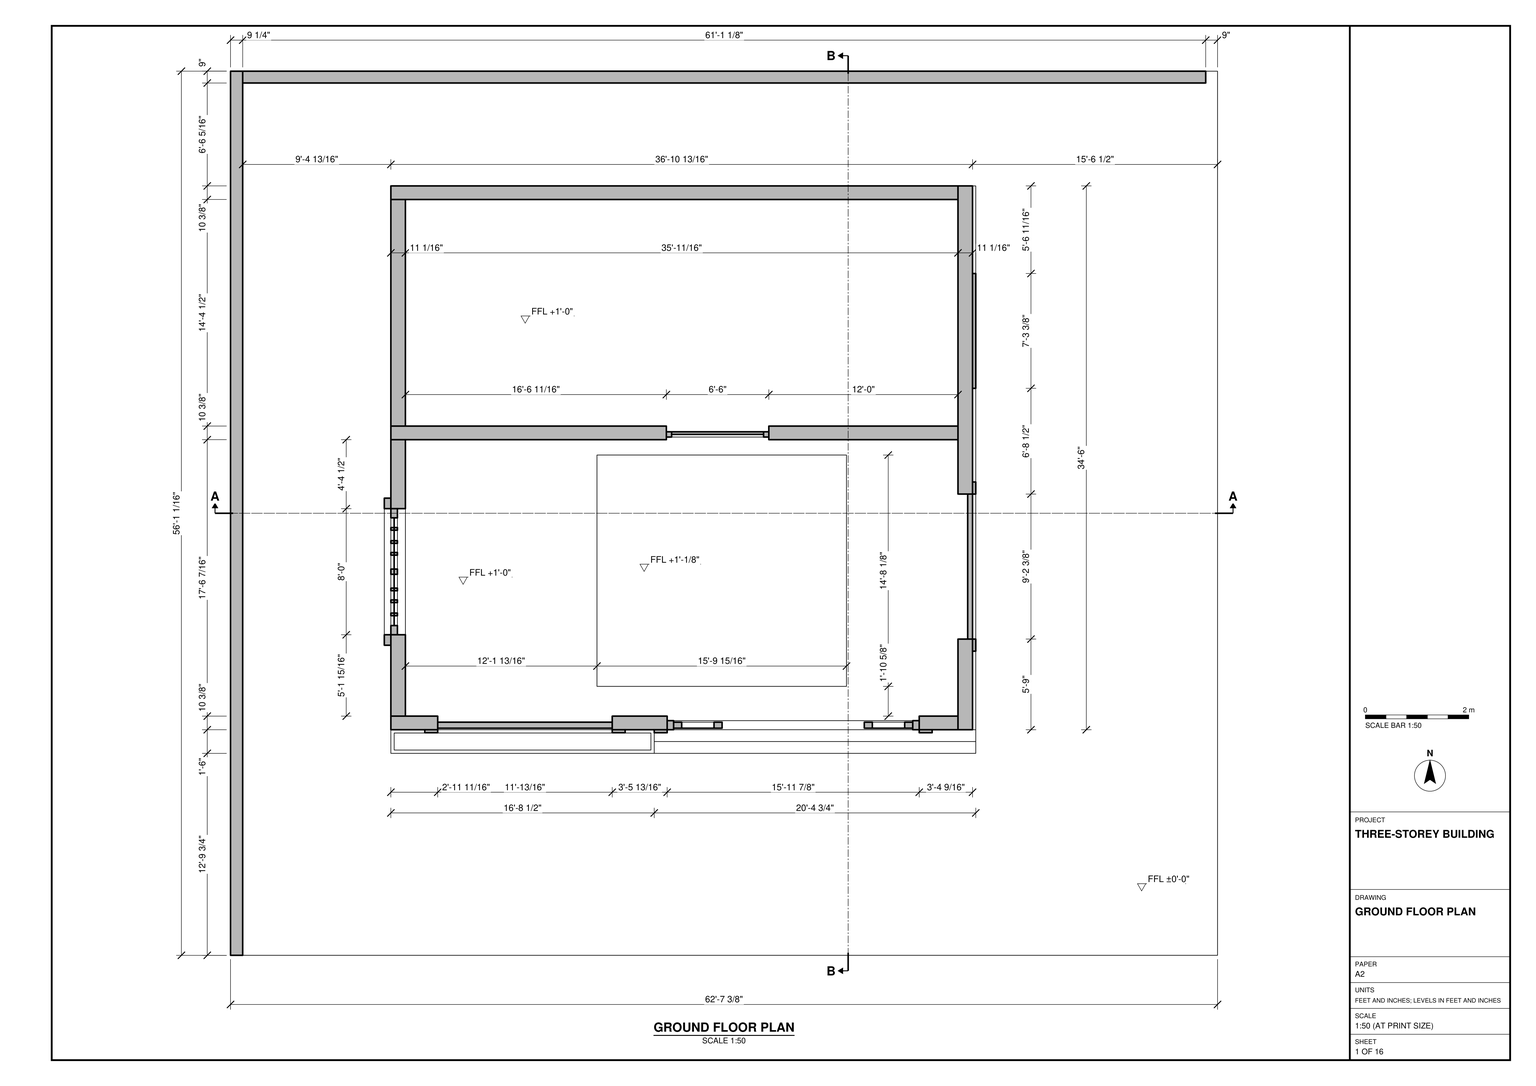
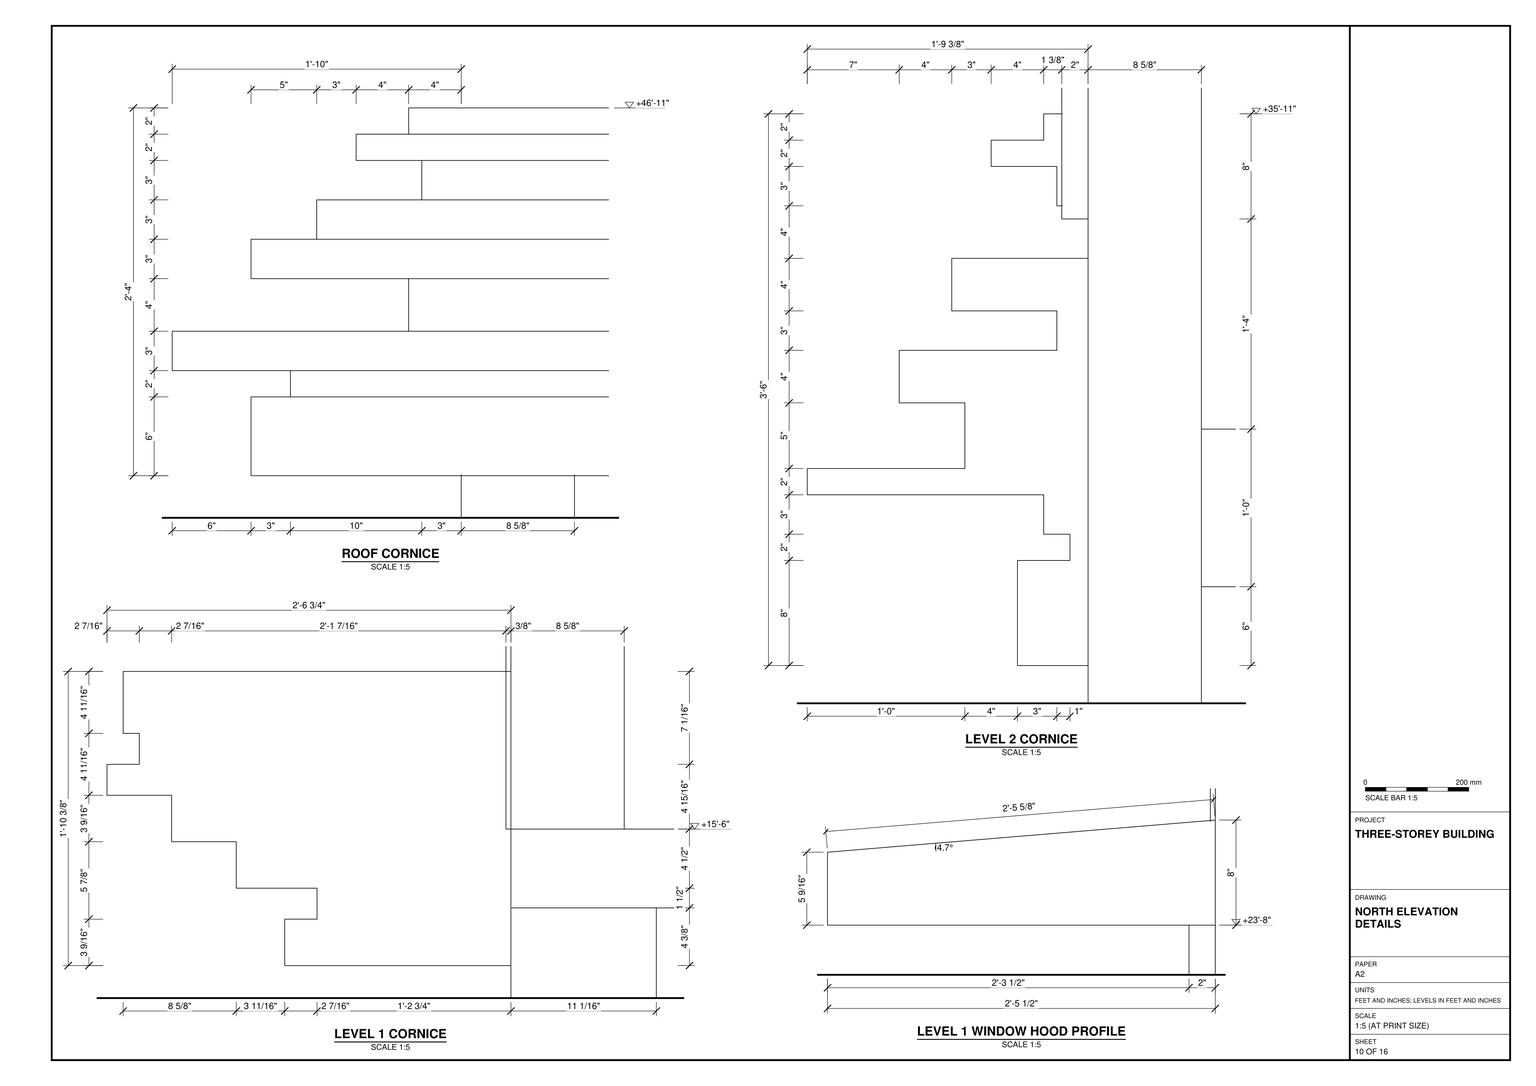
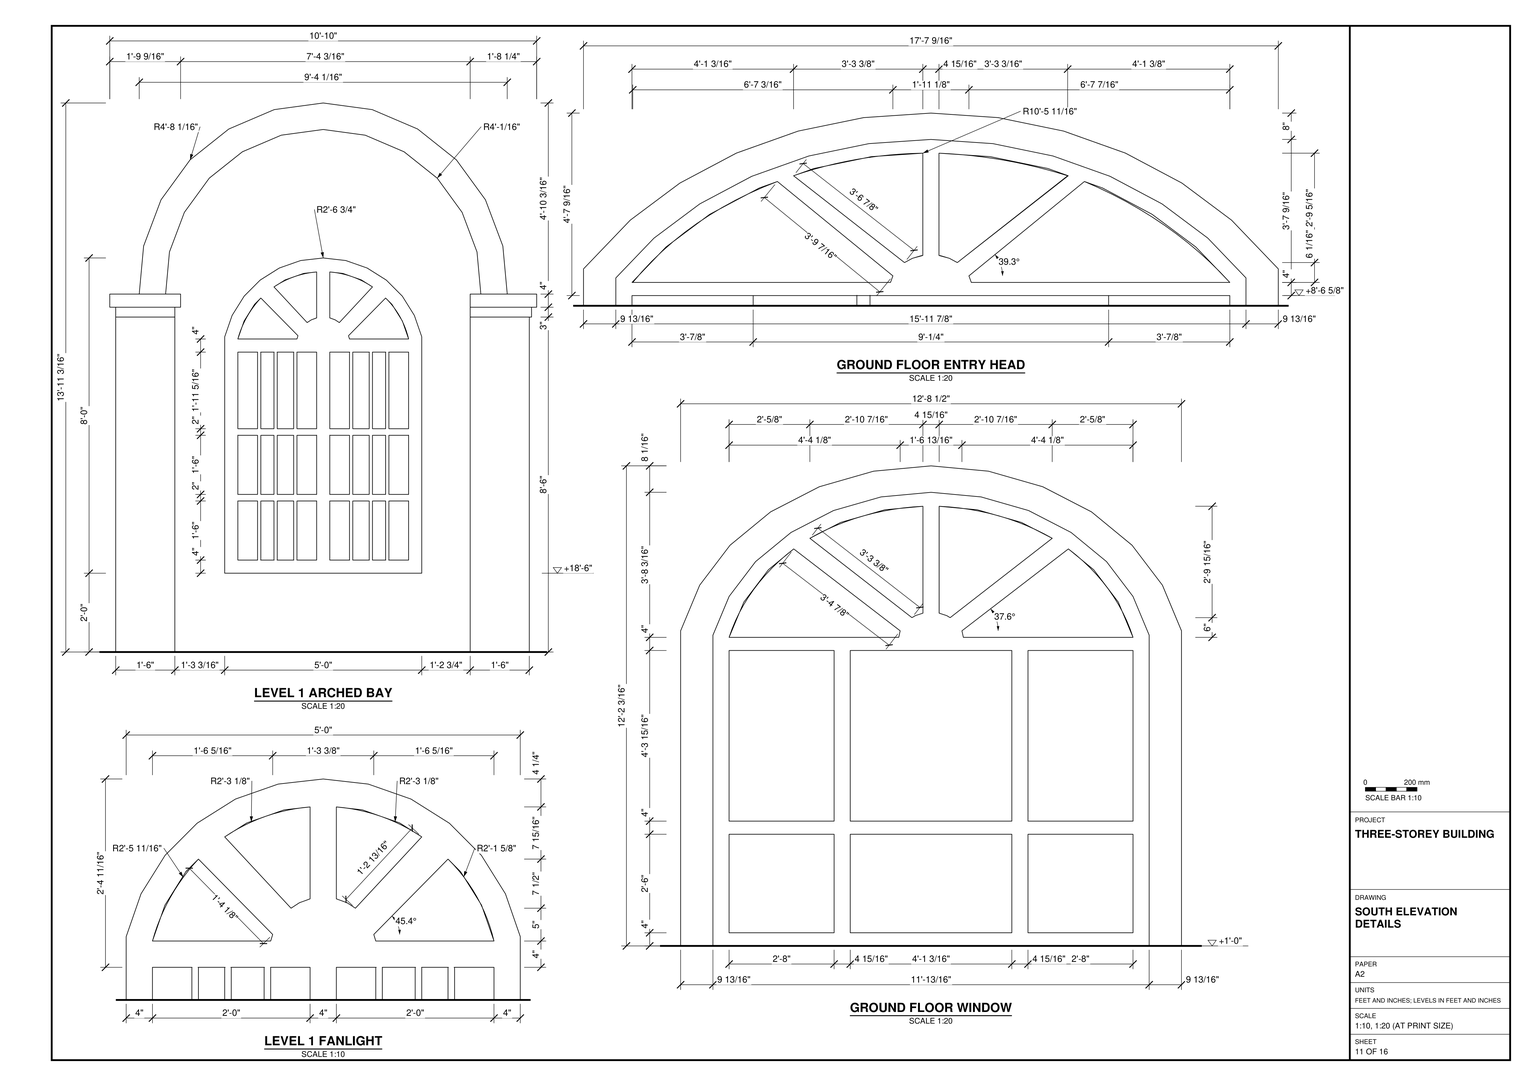
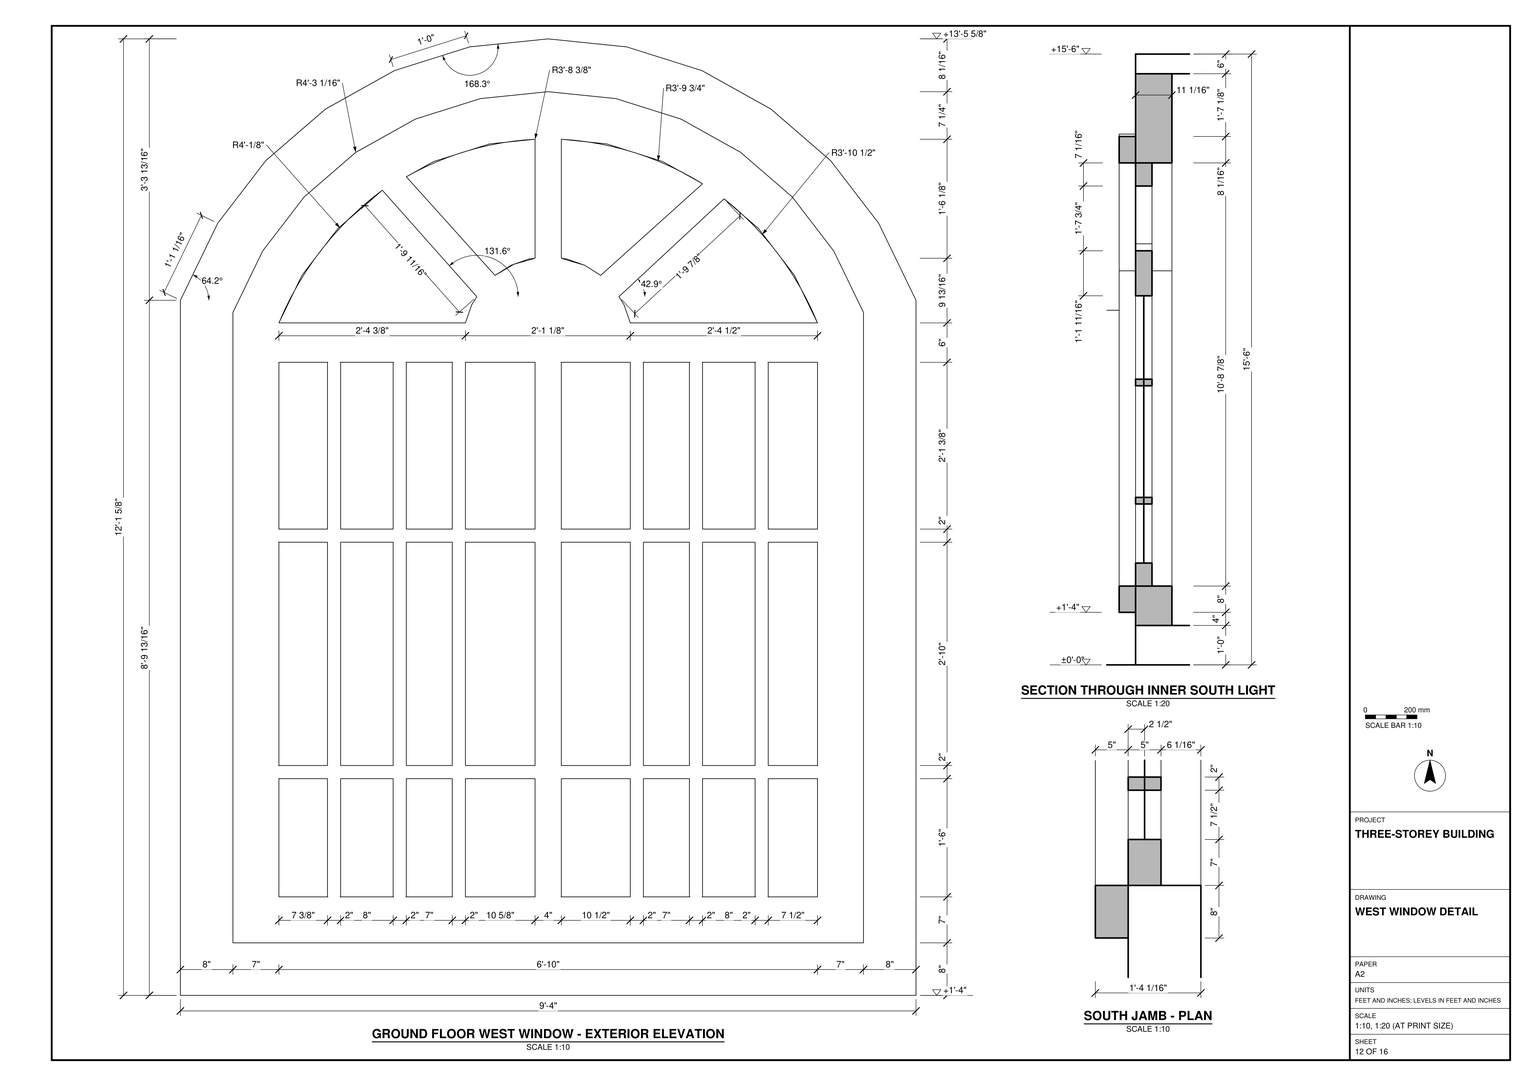
Build the three-storey building and its site in SketchUp from task_files/diagram_01.pdf. Work in feet and inches. The overall model, including the site, measures 62'-7 3/8" along X, 56'-1 1/16" along Y and 47'-5" along Z. Use the reference levels ±0'-0", +15'-6" and +35'-11". Distinguish the site datum from the raised ground-floor finish shown on the plan.

Set out the building relative to the north and west boundary walls, retaining the setbacks on the plan. Model the floor slabs, exterior walls, internal partitions and roof to the profiles and thicknesses drawn. On the ground floor, place the transverse partition and its opening between the front and rear spaces. Use the elevations and enlarged details together to form the south entrance head, the adjacent arched window and the upper arched bays. Give the window frames, fanlights, hoods and cornices their drawn depth rather than representing them with lines on the facade. Follow the sheets for any stairs, built-in joinery and main furniture shown. Decor and loose items may be any suitable library components placed where indicated.

Keep shell elements such as walls, slabs and roof, and each furniture or joinery piece, in separate groups or components. Use components for repeated parts. Save one SketchUp model as output_files/three_storey_building_with_arched_bays_and_cornices.skp.

# SketchUp Ruby script. Lengths in inches.
U = 1.inch
M = Sketchup.active_model
def pt(a) = Geom::Point3d.new(a.map { |v| v * U })
def face(e, loops, mat)
  f = e.add_face(loops[0].map { |a| pt(a) })
  loops[1..].each { |l| e.add_face(l.map { |a| pt(a) }).erase! }
  f.material = f.back_material = mat if mat
  f
end
# faces: each face lists its corners as indices into pts; further lists are holes
def faces(e, pts, list, mat = nil) = list.each { |f| face(e, (f[0].is_a?(Array) ? f : [f]).map { |l| l.map { |i| pts[i] } }, mat) }
# xy, xz, yz: faces in a plane at the given z, y or x. An outline is a flat list of corners, or four numbers for a rectangle; further outlines are holes
def ring(l) = l.size == 4 ? [[l[0], l[1]], [l[2], l[1]], [l[2], l[3]], [l[0], l[3]]] : l.each_slice(2).to_a
def flat(e, list, mat, &to3) = list.each { |f| face(e, (f[0].is_a?(Array) ? f : [f]).map { |l| ring(l).map { |u, v| to3.(u, v) } }, mat) }
def xy(e, z, list, mat = nil) = flat(e, list, mat) { |x, y| [x, y, z] }
def xz(e, y, list, mat = nil) = flat(e, list, mat) { |x, z| [x, y, z] }
def yz(e, x, list, mat = nil) = flat(e, list, mat) { |y, z| [x, y, z] }
def lines(e, pts, list) = list.each { |a, b| e.add_line(pt(pts[a]), pt(pts[b])) }
# prism: a flat outline (further loops are holes) pulled along v
def prism(e, loops, v, mat = nil)
  f = face(e, loops, mat); d = Geom::Vector3d.new(v.map { |x| x * U })
  f.pushpull(f.normal.samedirection?(d) ? d.length : -d.length)
end
def box(e, o, s, mat = nil) = prism(e, [[o, [o[0] + s[0], o[1], o[2]], [o[0] + s[0], o[1] + s[1], o[2]], [o[0], o[1] + s[1], o[2]]]], [0, 0, s[2]], mat)
def at(x, y, z, deg = 0) = Geom::Transformation.translation(pt([x, y, z])) * Geom::Transformation.rotation(ORIGIN, Z_AXIS, deg.degrees)
def axes(o, x, y, z) = Geom::Transformation.new([*x, 0, *y, 0, *z, 0, *pt(o).to_a, 1])
def part(name) = M.definitions.add(name)
# library, detail: a bought-in or finely detailed component or shape, given as its bounding box
def library(name, o, s) = part(name).tap { |d| box(d.entities, o, s) }
def detail(e, o, s) = box(e.add_group.entities, o, s)
def put(e, d, t, mat = nil) = e.add_instance(d, t).tap { |i| i.material = mat if mat }
def group(e, t, mat = nil) = e.add_group.tap { |g| g.transformation = t; g.material = mat if mat }.entities
root = M.entities
M.materials.add("[Color C02]").color = [255, 204, 153]
M.materials.add("[Color C06]").color = [204, 102, 0]
M.materials.add("[Color M07]").color = [58, 58, 58]
M.materials.add("[Grass Dark Green]").color = [106, 157, 55]
M.materials.add("[Leather Red Brown]").color = [76, 40, 8]
M.materials.add("[Metal Silver]").color = [234, 233, 238]
M.materials.add("[Slate Light Tile]").color = [54, 54, 54]
M.materials.add("[Tile Various Tan]").color = [214, 196, 169]
M.materials.add("[Translucent Glass Gray]").color = [147, 147, 147]
M.materials["[Translucent Glass Gray]"].alpha = 0.5
M.materials.add("[Wood Veneer 01]").color = [120, 70, 37]
c1 = library("Group\#4",[0,0,8],[2,112,138.17])
c2 = part("Group\#10")
prism(c2.entities,[[[0,78,0],[0,78,8],[24,78,5.56],[24,78,0]]],[0,-78,0])
c3 = library("Group\#11",[0,0,0],[3,96,130.125])
c4 = library("Group\#31",[0,0,8],[172,2,146.19])
c5 = library("Group\#32",[0,0,0],[156,6,138.17])
c6 = library("Group\#27",[0,0,8],[124,2,146.1875])
c7 = library("Group\#41",[0,0,0],[108,4,138.14])
c8 = part("Group\#56")
box(c8.entities,[0,0,0],[24,24,114])
c9 = library("Group\#59",[0,0,0],[60,3,96])
c10 = part("Group\#71")
box(c10.entities,[0,0,0],[28,26,3])
c11 = part("Group\#70")
box(c11.entities,[0,0,0],[36,30,4])
c12 = library("Group\#74",[0,0,0],[6.15,82.8,60])
c13 = part("Group\#73")
prism(c13.entities,[[[2,0,64],[2,0,0],[2,86.8,0],[2,86.8,64]],[[2,84.8,2],[2,2,2],[2,2,62],[2,84.8,62]]],[-2,0,0])
c14 = library("Group\#78",[0,0,0],[2.75,2.75,40.8125])
c15 = library("Group\#79",[0,0,0],[3.75,151.87,3.75])
c16 = library("Group\#97",[0,0,0],[5,112,145.64])
c17 = library("Group\#98",[0,0,0],[5,96,129.6])
c18 = library("Group\#107",[0,0,-121],[112.07,22.8,179.2])
g1 = group(root,at(38.125,77.25,0),"[Tile Various Tan]")
box(g1,[-38.125,-77.25,0],[751.36,673.09,6])
g2 = group(root,at(122.05,171.76,6))
xy(g2,0,[[0,0,445.26,414]])
xy(g2,12,[[0,0,445.26,414]])
xz(g2,0,[[0,0,445.26,12]],"[Color C06]")
xz(g2,414,[[0,0,445.26,12]],"[Color C06]")
yz(g2,0,[[0,0,414,12]],"[Color C06]")
yz(g2,445.26,[[0,0,414,12]],"[Color C06]")
g3 = group(root,at(553.78,171.76,18),"[Color C02]")
prism(g3,[[[11.07,69,0],[11.07,69,96],[11.07,74.09,105.47],[11.07,81.31,113.82],[11.07,90.34,120.72],[11.07,100.8,125.87],[11.07,112.24,129.05],[11.07,124.2,130.125],[11.07,136.16,129.05],[11.07,147.6,125.87],[11.07,158.0625,120.72],[11.07,167.09,113.82],[11.07,174.31,105.47],[11.07,179.4,96],[11.07,179.4,0],[11.07,414,0],[11.07,414,168],[11.07,0,168],[11.07,0,0]],[[11.07,262.2,96],[11.07,345,96],[11.07,345,36],[11.07,262.2,36]]],[-11.07,0,0])
put(root,c1,axes([564.85,231.56,10],[1.23,0,0],[0,1.15,0],[0,0,1]),"[Color C06]")
g4 = group(root,at(564.85,431.66,52),"[Color C06]")
prism(g4,[[[0,87.4,0],[0,0,0],[0,0,64],[0,87.4,64]],[[0,85.1,62],[0,2.3,62],[0,2.3,2],[0,85.1,2]]],[2.46,0,0])
g5 = group(root,at(564.85,438.56,58),"[Translucent Glass Gray]")
yz(g5,0,[[0,0,73.6,52]])
put(root,c2,axes([564.85,430.51,116],[1.23,0,0],[0,1.15,0],[0,0,1]),"[Color C06]")
put(root,c3,axes([561.16,240.76,18],[1.23,0,0],[0,1.15,0],[0,0,1]),"[Wood Veneer 01]")
g6 = group(root,at(564.85,245.36,113.11),"[Translucent Glass Gray]")
yz(g6,0,[[0,0,1.05,2.41,2.25,4.75,3.61,7.04,5.11,9.25,6.77,11.38,8.56,13.43,10.48,15.38,12.53,17.24,14.7,18.99,16.98,20.62,19.37,22.14,21.85,23.53,48.3,0]])
g7 = group(root,at(564.85,271.81,117.11),"[Translucent Glass Gray]")
yz(g7,0,[[21.85,0,0,21.8,1.71,22.52,3.44,23.18,5.2,23.79,6.99,24.35,8.79,24.85,10.62,25.3,12.46,25.69,14.32,26.03,16.19,26.3,18.07,26.52,19.96,26.68,21.85,26.79]])
g8 = group(root,at(564.85,298.26,117.11),"[Translucent Glass Gray]")
yz(g8,0,[[0,0,0,26.79,1.88,26.61,3.75,26.39,5.62,26.13,7.48,25.82,9.32,25.47,11.16,25.07,12.98,24.63,14.79,24.15,16.58,23.625,18.36,23.06,20.11,22.45,21.85,21.8]])
g9 = group(root,at(564.85,298.26,113.11),"[Translucent Glass Gray]")
yz(g9,0,[[0,0,26.45,23.53,28.86,22.07,31.1875,20.5,33.42,18.82,35.54,17.05,37.5625,15.1875,39.47,13.24,41.26,11.21,42.93,9.1,44.47,6.91,45.88,4.67,47.16,2.36,48.3,0]])
g10 = group(root,at(564.85,245.36,56),"[Translucent Glass Gray]")
yz(g10,0,[[0,0,21.85,53.11]])
g11 = group(root,at(564.85,271.81,56),"[Translucent Glass Gray]")
yz(g11,0,[[0,0,21.85,53.11]])
g12 = group(root,at(564.85,298.26,56),"[Translucent Glass Gray]")
yz(g12,0,[[0,0,21.85,53.11]])
g13 = group(root,at(564.85,324.71,56),"[Translucent Glass Gray]")
yz(g13,0,[[0,0,21.85,53.11]])
g14 = group(root,at(564.85,245.36,22),"[Translucent Glass Gray]")
yz(g14,0,[[0,0,21.85,30]])
g15 = group(root,at(564.85,271.81,22),"[Translucent Glass Gray]")
yz(g15,0,[[0,0,21.85,30]])
g16 = group(root,at(564.85,298.26,22),"[Translucent Glass Gray]")
yz(g16,0,[[0,0,21.85,30]])
g17 = group(root,at(564.85,324.71,22),"[Translucent Glass Gray]")
yz(g17,0,[[0,0,21.85,30]])
g18 = group(root,at(122.05,575.41,18),"[Color C02]")
box(g18,[0,0,0],[431.73,10.35,168])
g19 = group(root,at(122.05,392.56,18),"[Color C02]")
prism(g19,[[[431.73,10.35,0],[287.73,10.35,0],[287.73,10.35,138],[209.73,10.35,138],[209.73,10.35,0],[0,10.35,0],[0,10.35,168],[431.73,10.35,168]]],[0,-10.35,0])
g20 = group(root,at(122.05,402.91,18),"[Color C02]")
box(g20,[0,0,0],[11.07,172.5,168])
g21 = group(root,at(122.05,171.76,186),"[Color C02]")
box(g21,[0,0,0],[442.8,414,6])
g22 = group(root,at(133.125,171.76,18),"[Color C02]")
prism(g22,[[[24.6,10.35,0],[-11.07,10.35,0],[-11.07,10.35,168],[420.66,10.35,168],[420.66,10.35,0],[391.14,10.35,0],[391.14,10.35,96],[379.51,10.35,108.13],[365.58,10.35,118.54],[349.73,10.35,126.95],[332.4,10.35,133.125],[314.06,10.35,136.9],[295.2,10.35,138.17],[276.34,10.35,136.9],[258,10.35,133.125],[240.67,10.35,126.95],[224.82,10.35,118.54],[210.89,10.35,108.13],[199.26,10.35,96],[199.26,10.35,0],[157.44,10.35,0],[157.44,10.35,94.625],[152.51,10.35,106.43],[144.45,10.35,117.04],[133.67,10.35,125.9],[120.72,10.35,132.58],[106.26,10.35,136.73],[91.02,10.35,138.14],[75.78,10.35,136.73],[61.32,10.35,132.58],[48.37,10.35,125.9],[37.59,10.35,117.04],[29.53,10.35,106.43],[24.6,10.35,94.625]]],[0,-10.35,0])
put(root,c4,axes([322.54,169.46,10],[1.23,0,0],[0,1.15,0],[0,0,1]),"[Color C06]")
put(root,c5,axes([332.38,171.76,18],[1.23,0,0],[0,1.15,0],[0,0,1]),"[Wood Veneer 01]")
g23 = group(root,at(337.3,172.91,22),"[Wood Veneer 01]")
prism(g23,[[[36.9,0,86.625],[0,0,86.625],[0,0,0],[36.9,0,0]],[[6.15,0,5],[6.15,0,81.625],[30.75,0,81.625],[30.75,0,5]]],[0,4.6,0])
g24 = group(root,at(482.44,172.91,22),"[Wood Veneer 01]")
prism(g24,[[[0,0,86.625],[0,0,0],[36.9,0,0],[36.9,0,86.625]],[[30.75,0,81.625],[30.75,0,5],[6.15,0,5],[6.15,0,81.625]]],[0,4.6,0])
g25 = group(root,at(337.53,171.76,112.625),"[Translucent Glass Gray]")
xz(g25,0,[[0,0,2.8,3.27,5.78,6.43,8.9375,9.47,12.27,12.4,15.75,15.19,19.4,17.86,23.1875,20.38,27.12,22.76,31.18,24.99,35.36,27.0625,39.65,28.98,44.05,30.73,79.21,2,78.49,0]])
g26 = group(root,at(386.5,171.76,118.67),"[Translucent Glass Gray]")
xz(g26,0,[[33.77,0,36.2,1.3,39.36,2.16,39.36,33.32,35.99,33.22,32.62,33.04,29.26,32.77,25.91,32.41,22.58,31.96,19.27,31.43,15.98,30.81,12.72,30.1,9.49,29.3125,6.29,28.4375,3.125,27.48,0,26.44]])
g27 = group(root,at(430.78,171.76,118.67),"[Translucent Glass Gray]")
xz(g27,0,[[5.59,0,3.16,1.3,0,2.16,0,33.32,3.35,33.14,6.6875,32.88,10.02,32.56,13.34,32.16,16.64,31.69,19.93,31.15,23.2,30.54,26.45,29.86,29.67,29.11,32.87,28.29,36.04,27.4,39.18,26.44]])
g28 = group(root,at(439.9,171.76,112.625),"[Translucent Glass Gray]")
xz(g28,0,[[0.72,0,0,2,35.16,30.73,39.47,28.84,43.68,26.82,47.8,24.67,51.8125,22.38,55.71,19.98,59.49,17.45,63.16,14.8125,66.6875,12.06,70.09,9.2,73.35,6.23,76.47,3.16,79.44,0]])
g29 = group(root,at(488.59,172.91,27),"[Translucent Glass Gray]")
xz(g29,0,[[0,0,24.6,76.625]])
g30 = group(root,at(343.45,172.91,27),"[Translucent Glass Gray]")
xz(g30,0,[[0,0,24.6,76.625]])
put(root,c6,axes([147.88,169.46,10],[1.23,0,0],[0,1.15,0],[0,0,1]),"[Color C06]")
put(root,c7,axes([157.72,172.91,18],[1.23,0,0],[0,1.15,0],[0,0,1]),"[Wood Veneer 01]")
g31 = group(root,at(162.64,172.91,111.96),"[Translucent Glass Gray]")
xz(g31,0,[[0,0,0.9,2.54,1.9375,5.05,3.12,7.51,4.45,9.93,5.91,12.29,7.5,14.59,9.23,16.84,11.08,19.01,13.06,21.11,15.15,23.13,17.36,25.08,19.68,26.93,52.09,2,51.66,0]])
g32 = group(root,at(187.24,172.91,117.96),"[Translucent Glass Gray]")
xz(g32,0,[[31.08,0,32.11,0.62,34.43,1.37,34.43,33.92,31.36,33.72,28.31,33.4,25.27,32.97,22.27,32.43,19.3,31.77,16.37,31.01,13.49,30.13,10.66,29.14,7.89,28.05,5.1875,26.86,2.56,25.5625,0,24.17]])
g33 = group(root,at(226.62,172.91,117.96),"[Translucent Glass Gray]")
xz(g33,0,[[3.34,0,2.32,0.62,0,1.37,0,33.92,3.07,33.73,6.125,33.42,9.16,32.99,12.16,32.45,15.13,31.79,18.0625,31.03,20.94,30.15,23.77,29.16,26.54,28.07,29.24,26.87,31.875,25.57,34.43,24.17]])
g34 = group(root,at(233.55,172.91,111.96),"[Translucent Glass Gray]")
xz(g34,0,[[0.43,0,52.09,0,51.21,2.55,50.18,5.06,49.01,7.52,47.6875,9.94,46.23,12.31,44.64,14.62,42.91,16.86,41.05,19.03,39.07,21.13,36.96,23.15,34.74,25.08,32.41,26.93,0,2]])
g35 = group(root,at(162.64,172.91,56),"[Translucent Glass Gray]")
xz(g35,0,[[0,0,31.98,51.96]])
g36 = group(root,at(199.54,172.91,56),"[Translucent Glass Gray]")
xz(g36,0,[[0,0,49.2,51.96]])
g37 = group(root,at(253.66,172.91,56),"[Translucent Glass Gray]")
xz(g37,0,[[0,0,31.98,51.96]])
g38 = group(root,at(162.64,172.91,22),"[Translucent Glass Gray]")
xz(g38,0,[[0,0,31.98,30]])
g39 = group(root,at(199.54,172.91,22),"[Translucent Glass Gray]")
xz(g39,0,[[0,0,49.2,30]])
g40 = group(root,at(253.66,172.91,22),"[Translucent Glass Gray]")
xz(g40,0,[[0,0,31.98,30]])
g41 = group(root,at(122.05,182.11,18),"[Color C02]")
prism(g41,[[[11.07,0,0],[11.07,210.45,0],[11.07,210.45,168],[11.07,0,168]],[[11.07,61.95,12],[11.07,61.95,108],[11.07,66.48,117.34],[11.07,72.8,125.58],[11.07,80.65,132.37],[11.07,89.72,137.42],[11.07,99.62,140.55],[11.07,109.95,141.6],[11.07,120.28,140.55],[11.07,130.18,137.42],[11.07,139.25,132.37],[11.07,147.1,125.58],[11.07,153.42,117.34],[11.07,157.95,108],[11.07,157.95,12]]],[-11.07,0,0])
g42 = group(root,at(107.22,143.01,181.61),"[Color C06]")
xy(g42,0,[[14.84,12.65,14.84,28.75,457.64,28.75,457.64,246.17,474.86,246.17,474.86,12.65]])
xy(g42,3.54,[[14.84,12.65,474.86,12.65,474.86,246.17,472.4,246.17,472.4,14.95,14.84,14.95]])
xy(g42,5.89,[[14.84,9.2,14.84,14.95,472.4,14.95,472.4,246.17,478.55,246.17,478.55,9.2]])
xy(g42,9.43,[[14.84,4.6,14.84,9.2,478.55,9.2,478.55,246.17,483.47,246.17,483.47,4.6]])
xy(g42,12.96,[[14.84,0,14.84,4.6,483.47,4.6,483.47,246.17,488.39,246.17,488.39,0]])
xy(g42,15.32,[[14.84,0,488.39,0,488.39,246.17,485.93,246.17,485.93,2.3,14.84,2.3]])
xy(g42,17.68,[[14.84,1.15,14.84,2.3,485.93,2.3,485.93,246.17,487.16,246.17,487.16,1.15]])
xy(g42,22.39,[[14.84,1.15,487.16,1.15,487.16,246.17,457.64,246.17,457.64,28.75,14.84,28.75]])
xz(g42,0,[[14.84,12.96,488.39,15.32]])
xz(g42,1.15,[[14.84,17.68,487.16,22.39]])
xz(g42,2.3,[[14.84,15.32,485.93,17.68]])
xz(g42,4.6,[[14.84,9.43,483.47,12.96]])
xz(g42,9.2,[[14.84,5.89,478.55,9.43]])
xz(g42,12.65,[[14.84,0,474.86,3.54]])
xz(g42,14.95,[[14.84,3.54,472.4,5.89]])
xz(g42,28.75,[[14.84,0,457.64,8.25],[14.84,8.25,457.64,22.39]])
xz(g42,246.17,[[457.64,0,457.64,22.39,487.16,22.39,487.16,17.68,485.93,17.68,485.93,15.32,488.39,15.32,488.39,12.96,483.47,12.96,483.47,9.43,478.55,9.43,478.55,5.89,472.4,5.89,472.4,3.54,474.86,3.54,474.86,0]])
yz(g42,14.84,[[12.65,0,12.65,3.54,14.95,3.54,14.95,5.89,9.2,5.89,9.2,9.43,4.6,9.43,4.6,12.96,0,12.96,0,15.32,2.3,15.32,2.3,17.68,1.15,17.68,1.15,22.39,28.75,22.39,28.75,0]])
yz(g42,457.64,[[28.75,0,246.17,8.25],[28.75,8.25,246.17,22.39]])
yz(g42,472.4,[[14.95,3.54,246.17,5.89]])
yz(g42,474.86,[[12.65,0,246.17,3.54]])
yz(g42,478.55,[[9.2,5.89,246.17,9.43]])
yz(g42,483.47,[[4.6,9.43,246.17,12.96]])
yz(g42,485.93,[[2.3,15.32,246.17,17.68]])
yz(g42,487.16,[[1.15,17.68,246.17,22.39]])
yz(g42,488.39,[[0,12.96,246.17,15.32]])
put(root,c8,axes([298.54,182.11,192],[1,0,0],[0,1.15,0],[0,0,1]),"[Color C02]")
g43 = group(root,at(289.54,209.71,192),"[Color C02]")
box(g43,[0,10.35,0],[9,172.5,209])
g44 = group(root,at(122.05,209.71,192),"[Color C02]")
prism(g44,[[[0,0,0],[176.49,0,0],[176.49,0,209],[0,0,209]],[[58.24,0,36],[58.24,0,108],[60.51,0,114.52],[64.16,0,120.37],[69.04,0,125.26],[74.875,0,128.94],[81.39,0,131.23],[88.24,0,132],[95.1,0,131.23],[101.62,0,128.94],[107.45,0,125.26],[112.33,0,120.37],[115.98,0,114.52],[118.24,0,108],[118.24,0,36]]],[0,10.35,0])
put(root,c9,axes([180.3,218.01,228],[1,0,0],[0,1.15,0],[0,0,1]),"[Wood Veneer 01]")
g45 = group(root,at(212.3,219.73,232),"[Translucent Glass Gray]")
xz(g45,0,[[0,0,24,63.33]])
g46 = group(root,at(184.3,219.73,232),"[Translucent Glass Gray]")
xz(g46,0,[[0,0,24,63.33]])
g47 = group(root,at(184.3,218.01,299.33),"[Translucent Glass Gray]")
xz(g47,0,[[0,0,0.34,1.15,0.73,2.29,1.16,3.42,1.64,4.52,2.17,5.61,2.74,6.67,3.35,7.71,4,8.72,4.69,9.7,5.42,10.66,6.19,11.58,7,12.48,18.3,1,18,0]])
g48 = group(root,at(195.3,218.01,304.33),"[Translucent Glass Gray]")
xz(g48,0,[[10.1,0,0,10.86,0.98,11.49,1.98,12.08,3,12.62,4.05,13.12,5.12,13.57,6.21,13.98,7.31,14.34,8.43,14.66,9.56,14.92,10.7,15.14,11.85,15.3,13,15.42,13,1.42,11.36,0.83]])
g49 = group(root,at(212.3,218.01,304.33),"[Translucent Glass Gray]")
xz(g49,0,[[2.9,0,1.64,0.83,0,1.42,0,15.42,1.15,15.3,2.3,15.14,3.44,14.92,4.57,14.66,5.69,14.34,6.79,13.98,7.88,13.57,8.95,13.12,10,12.62,11.02,12.08,12.02,11.49,13,10.86]])
g50 = group(root,at(218,218.01,299.33),"[Translucent Glass Gray]")
xz(g50,0,[[0.3,0,0,1,11.3,12.48,12.14,11.61,12.94,10.71,13.7,9.76,14.41,8.79,15.08,7.78,15.69,6.74,16.26,5.67,16.77,4.58,17.24,3.46,17.65,2.32,18,1.17,18.3,0]])
g51 = group(root,at(298.54,180.96,317),"[Color C02]")
xy(g51,-4,[[11.48,-5.75,11.48,0,0,0,0,28.75,24,28.75,24,-5.75],[235.56,-5.75,235.56,27.375,266.31,27.375,266.31,0,248.08,0,248.08,-5.75]])
xy(g51,0,[[235.56,27.375,244.46,28.75]])
xy(g51,84,[[0,0,266.31,0,266.31,27.375,244.46,27.375,244.46,28.75,0,28.75]])
xz(g51,-5.75,[[11.48,-4,24,-4,24,0,38.9375,12.4,55.32,22.83,72.875,31.12,91.33,37.13,110.4,40.78,129.78,42,149.16,40.78,168.23,37.13,186.6875,31.12,204.24,22.83,220.62,12.4,235.56,0,235.56,-4,248.08,-4,248.08,0,225.34,18.88,208.12,29.85,189.64,38.57,170.22,44.89,150.16,48.73,129.78,50.02,109.4,48.73,89.34,44.89,69.92,38.57,51.44,29.85,34.22,18.88,11.48,0]],"[Color C06]")
xz(g51,0,[[0,-4,11.48,-4,11.48,0,34.22,18.88,51.44,29.85,69.92,38.57,89.34,44.89,109.4,48.73,129.78,50.02,150.16,48.73,170.22,44.89,189.64,38.57,208.12,29.85,225.34,18.88,248.08,0,248.08,-4,266.31,-4,266.31,84,0,84]])
xz(g51,27.375,[[235.56,-4,235.56,0,244.46,0,244.46,84,266.31,84,266.31,-4]])
xz(g51,28.75,[[0,-4,0,84,244.46,84,244.46,0,235.56,0,220.62,12.4,204.24,22.83,186.6875,31.12,168.23,37.13,149.16,40.78,129.78,42,110.4,40.78,91.33,37.13,72.875,31.12,55.32,22.83,38.9375,12.4,24,0,24,-4]])
yz(g51,0,[[0,-4,28.75,84]])
yz(g51,11.48,[[-5.75,-4,0,0]],"[Color C06]")
yz(g51,24,[[-5.75,-4,28.75,0]],"[Color C06]")
yz(g51,235.56,[[-5.75,-4,27.375,0]],"[Color C06]")
yz(g51,244.46,[[27.375,0,28.75,84]])
yz(g51,248.08,[[-5.75,-4,0,0]],"[Color C06]")
yz(g51,266.31,[[0,-4,27.375,84]])
p = [[34.22,0,18.88],[11.48,0,0],[11.48,-5.75,0],[34.22,-5.75,18.88],[38.9375,28.75,12.4],[38.9375,-5.75,12.4],
  [24,-5.75,0],[24,28.75,0],[235.56,27.375,0],[235.56,-5.75,0],[220.62,-5.75,12.4],[220.62,28.75,12.4],
  [235.56,28.75,0],[248.08,0,0],[225.34,0,18.88],[225.34,-5.75,18.88],[248.08,-5.75,0],[55.32,28.75,22.83],
  [55.32,-5.75,22.83],[204.24,-5.75,22.83],[204.24,28.75,22.83],[51.44,0,29.85],[51.44,-5.75,29.85],[208.12,0,29.85],
  [208.12,-5.75,29.85],[72.875,28.75,31.12],[72.875,-5.75,31.12],[186.6875,-5.75,31.12],[186.6875,28.75,31.12],[69.92,0,38.57],
  [69.92,-5.75,38.57],[189.64,0,38.57],[189.64,-5.75,38.57],[91.33,28.75,37.13],[91.33,-5.75,37.13],[168.23,-5.75,37.13],
  [168.23,28.75,37.13],[110.4,28.75,40.78],[110.4,-5.75,40.78],[149.16,-5.75,40.78],[149.16,28.75,40.78],[89.34,0,44.89],
  [89.34,-5.75,44.89],[170.22,0,44.89],[170.22,-5.75,44.89],[129.78,28.75,42],[129.78,-5.75,42],[109.4,0,48.73],
  [109.4,-5.75,48.73],[150.16,0,48.73],[150.16,-5.75,48.73],[129.78,0,50.02],[129.78,-5.75,50.02]]
faces(g51,p,[[0,1,2,3],[4,5,6,7],[8,9,10,11,12],[13,14,15,16],[17,18,5,4],[11,10,19,20],[21,0,3,22],[14,23,24,15],
  [25,26,18,17],[20,19,27,28],[29,21,22,30],[23,31,32,24],[33,34,26,25],[28,27,35,36],[37,38,34,33],[36,35,39,40],
  [41,29,30,42],[31,43,44,32],[45,46,38,37],[40,39,46,45],[47,41,42,48],[43,49,50,44],[51,47,48,52],[49,51,52,50]],"[Color C06]")
put(root,c10,axes([296.54,179.81,306],[1,0,0],[0,1.15,0],[0,0,1]),"[Color C06]")
put(root,c11,axes([292.54,175.21,309],[1,0,0],[0,1.15,0],[0,0,1]),"[Color C06]")
g52 = group(root,at(535.23,175.21,309),"[Color C06]")
box(g52,[0,0,0],[36,38.5,4])
g53 = group(root,at(539.23,179.81,306),"[Color C06]")
box(g53,[0,0,0],[28,31.9,3])
g54 = group(root,at(541.23,182.11,192),"[Color C02]")
box(g54,[0,0,0],[24,27.6,114])
put(root,c11,axes([535.23,354.68,309],[1,0,0],[0,1.15,0],[0,0,1]),"[Color C06]")
put(root,c8,axes([541.23,361.58,192],[1,0,0],[0,1.15,0],[0,0,1]),"[Color C02]")
put(root,c10,axes([539.23,359.28,306],[1,0,0],[0,1.15,0],[0,0,1]),"[Color C06]")
g55 = group(root,at(564.85,193.24,317),"[Color C02]")
xy(g55,-4,[[-21.85,0,-21.85,16.32,5.75,16.32,5.75,7.8,0,7.8,0,0],[-21.85,160.18,-21.85,195.93,0,195.93,0,168.7,5.75,168.7,5.75,160.18]])
xy(g55,84,[[-21.85,0,0,195.93]])
xz(g55,0,[[-21.85,-4,-6.75,84],[-6.75,-4,0,84]])
xz(g55,7.8,[[0,-4,5.75,0]],"[Color C06]")
xz(g55,16.32,[[-21.85,-4,5.75,0]],"[Color C06]")
xz(g55,160.18,[[-21.85,-4,5.75,0]],"[Color C06]")
xz(g55,168.7,[[0,-4,5.75,0]],"[Color C06]")
xz(g55,195.93,[[-21.85,-4,0,84]])
yz(g55,-21.85,[[0,-4,0,84,195.93,84,195.93,-4,160.18,-4,160.18,0,150.02,12.4,138.89,22.83,126.95,31.12,114.39,37.13,101.43,40.78,88.25,42,75.07,40.78,62.11,37.13,49.55,31.12,37.61,22.83,26.48,12.4,16.32,0,16.32,-4]])
yz(g55,0,[[0,-4,7.8,-4,7.8,0,23.27,18.88,34.98,29.85,47.54,38.57,60.75,44.89,74.39,48.73,88.25,50.02,102.11,48.73,115.75,44.89,128.96,38.57,141.52,29.85,153.23,18.88,168.7,0,168.7,-4,195.93,-4,195.93,84,0,84]])
yz(g55,5.75,[[7.8,-4,16.32,-4,16.32,0,26.48,12.4,37.61,22.83,49.55,31.12,62.11,37.13,75.07,40.78,88.25,42,101.43,40.78,114.39,37.13,126.95,31.12,138.89,22.83,150.02,12.4,160.18,0,160.18,-4,168.7,-4,168.7,0,153.23,18.88,141.52,29.85,128.96,38.57,115.75,44.89,102.11,48.73,88.25,50.02,74.39,48.73,60.75,44.89,47.54,38.57,34.98,29.85,23.27,18.88,7.8,0]],"[Color C06]")
p = [[0,23.27,18.88],[0,7.8,0],[5.75,7.8,0],[5.75,23.27,18.88],[-21.85,26.48,12.4],[5.75,26.48,12.4],
  [5.75,16.32,0],[-21.85,16.32,0],[-21.85,160.18,0],[5.75,160.18,0],[5.75,150.02,12.4],[-21.85,150.02,12.4],
  [0,168.7,0],[0,153.23,18.88],[5.75,153.23,18.88],[5.75,168.7,0],[-21.85,37.61,22.83],[5.75,37.61,22.83],
  [5.75,138.89,22.83],[-21.85,138.89,22.83],[0,34.98,29.85],[5.75,34.98,29.85],[0,141.52,29.85],[5.75,141.52,29.85],
  [-21.85,49.55,31.12],[5.75,49.55,31.12],[5.75,126.95,31.12],[-21.85,126.95,31.12],[0,47.54,38.57],[5.75,47.54,38.57],
  [0,128.96,38.57],[5.75,128.96,38.57],[-21.85,62.11,37.13],[5.75,62.11,37.13],[5.75,114.39,37.13],[-21.85,114.39,37.13],
  [-21.85,75.07,40.78],[5.75,75.07,40.78],[5.75,101.43,40.78],[-21.85,101.43,40.78],[0,60.75,44.89],[5.75,60.75,44.89],
  [0,115.75,44.89],[5.75,115.75,44.89],[-21.85,88.25,42],[5.75,88.25,42],[0,74.39,48.73],[5.75,74.39,48.73],
  [0,102.11,48.73],[5.75,102.11,48.73],[0,88.25,50.02],[5.75,88.25,50.02]]
faces(g55,p,[[0,1,2,3],[4,5,6,7],[8,9,10,11],[12,13,14,15],[16,17,5,4],[11,10,18,19],[20,0,3,21],[13,22,23,14],
  [24,25,17,16],[19,18,26,27],[28,20,21,29],[22,30,31,23],[32,33,25,24],[27,26,34,35],[36,37,33,32],[35,34,38,39],
  [40,28,29,41],[30,42,43,31],[44,45,37,36],[39,38,45,44],[46,40,41,47],[42,48,49,43],[50,46,47,51],[48,50,51,49]],"[Color C06]")
g56 = group(root,at(556.23,389.18,192),"[Color C02]")
prism(g56,[[[0,196.58,0],[0,0,0],[0,0,353],[0,196.58,353]],[[0,45.08,96],[0,45.08,36],[0,127.88,36],[0,127.88,96]],[[0,127.88,299],[0,45.08,299],[0,45.08,239],[0,127.88,239]]],[8.62,0,0])
put(root,c12,at(558.7,433.96,54),"[Wood Veneer 01]")
put(root,c12,at(558.7,434.26,228),"[Wood Veneer 01]")
put(root,c13,at(564.85,432.26,226),"[Color C06]")
g57 = group(root,at(564.85,438.86,232),"[Translucent Glass Gray]")
yz(g57,0,[[0,0,73.6,52]])
put(root,c2,axes([564.85,430.51,290],[1.23,0,0],[0,1.15,0],[0,0,1]),"[Color C06]")
g58 = group(root,at(298.54,389.18,192),"[Color C02]")
prism(g58,[[[27.6,9,0],[0,9,0],[0,9,209],[257.6875,9,209],[257.6875,9,0],[87.6,9,0],[87.6,9,120],[27.6,9,120]]],[0,-9,0])
g59 = group(root,at(322.54,182.11,192),"[Color C02]")
box(g59,[0,0,0],[218.6875,27.6,20])
g60 = group(root,at(322.54,194.28,250.375),"[Wood Veneer 01]")
prism(g60,[[[0,0.48,0.48],[0,0.22,0.8125],[0,0.06,1.2],[0,0,1.625],[0,0.06,2.05],[0,0.22,2.4375],[0,0.48,2.77],[0,0.8125,3.03],[0,1.2,3.19],[0,1.625,3.25],[0,2.05,3.19],[0,2.4375,3.03],[0,2.77,2.77],[0,3.03,2.4375],[0,3.19,2.05],[0,3.25,1.625],[0,3.19,1.2],[0,3.03,0.8125],[0,2.77,0.48],[0,2.4375,0.22],[0,2.05,0.06],[0,1.625,0],[0,1.2,0.06],[0,0.8125,0.22]]],[218.6875,0,0])
put(root,c14,at(326.94,194.53,212),"[Wood Veneer 01]")
put(root,c14,at(336.94,194.53,212),"[Wood Veneer 01]")
put(root,c14,at(346.94,194.53,212),"[Wood Veneer 01]")
put(root,c14,at(356.94,194.53,212),"[Wood Veneer 01]")
put(root,c14,at(366.94,194.53,212),"[Wood Veneer 01]")
put(root,c14,at(376.94,194.53,212),"[Wood Veneer 01]")
put(root,c14,at(386.94,194.53,212),"[Wood Veneer 01]")
put(root,c14,at(396.94,194.53,212),"[Wood Veneer 01]")
put(root,c14,at(406.94,194.53,212),"[Wood Veneer 01]")
put(root,c14,at(416.94,194.53,212),"[Wood Veneer 01]")
put(root,c14,at(426.94,194.53,212),"[Wood Veneer 01]")
put(root,c14,at(436.94,194.53,212),"[Wood Veneer 01]")
put(root,c14,at(446.94,194.53,212),"[Wood Veneer 01]")
put(root,c14,at(456.94,194.53,212),"[Wood Veneer 01]")
put(root,c14,at(466.94,194.53,212),"[Wood Veneer 01]")
put(root,c14,at(476.94,194.53,212),"[Wood Veneer 01]")
put(root,c14,at(486.94,194.53,212),"[Wood Veneer 01]")
put(root,c14,at(496.94,194.53,212),"[Wood Veneer 01]")
put(root,c14,at(506.94,194.53,212),"[Wood Veneer 01]")
put(root,c14,at(516.94,194.53,212),"[Wood Veneer 01]")
put(root,c14,at(526.94,194.53,212),"[Wood Veneer 01]")
g61 = group(root,at(541.23,209.71,192),"[Color C02]")
box(g61,[0,0,0],[24,151.87,20])
put(root,c15,at(551.36,209.71,250.125),"[Wood Veneer 01]")
put(root,c14,at(551.97,214.87,212.2),"[Wood Veneer 01]")
put(root,c14,at(551.97,224.87,212.2),"[Wood Veneer 01]")
put(root,c14,at(551.97,234.87,212.2),"[Wood Veneer 01]")
put(root,c14,at(551.97,244.87,212.2),"[Wood Veneer 01]")
put(root,c14,at(551.97,254.87,212.2),"[Wood Veneer 01]")
put(root,c14,at(551.97,264.87,212.2),"[Wood Veneer 01]")
put(root,c14,at(551.97,274.87,212.2),"[Wood Veneer 01]")
put(root,c14,at(551.97,284.87,212.2),"[Wood Veneer 01]")
put(root,c14,at(551.97,294.87,212.2),"[Wood Veneer 01]")
put(root,c14,at(551.97,304.87,212.2),"[Wood Veneer 01]")
put(root,c14,at(551.97,314.87,212.2),"[Wood Veneer 01]")
put(root,c14,at(551.97,324.87,212.2),"[Wood Veneer 01]")
put(root,c14,at(551.97,334.87,212.2),"[Wood Veneer 01]")
put(root,c14,at(551.97,344.87,212.2),"[Wood Veneer 01]")
put(root,c14,at(551.97,354.87,212.2),"[Wood Veneer 01]")
g62 = group(root,at(122.05,220.06,192),"[Color C02]")
box(g62,[0,0,0],[9,365.7,209])
g63 = group(root,at(131.05,576.76,192),"[Color C02]")
box(g63,[0,0,0],[425.18,9,209])
g64 = group(root,at(564.85,438.86,435),"[Translucent Glass Gray]")
yz(g64,0,[[0,0,73.6,52]])
g65 = group(root,at(122.05,189.58,401),"[Color C02]")
xy(g65,0,[[0,0,434.18,396.17]])
xy(g65,12,[[254.18,199.6,434.18,396.17]])
xy(g65,36,[[0,0,434.18,0,434.18,199.6,254.18,199.6,254.18,396.17,0,396.17]])
xz(g65,0,[[0,0,434.18,36]])
xz(g65,199.6,[[254.18,12,434.18,36]])
xz(g65,396.17,[[0,0,0,36,254.18,36,254.18,12,434.18,12,434.18,0]])
yz(g65,0,[[0,0,396.17,36]])
yz(g65,254.18,[[199.6,12,396.17,36]])
yz(g65,434.18,[[0,0,396.17,0,396.17,12,199.6,12,199.6,36,0,36]])
p = [[274.16,153.22,0],[254.18,199.6,36]]
lines(g65,p,[[0,1]])
g66 = group(root,at(376.23,576.76,413),"[Color C02]")
box(g66,[0,0,0],[180,9,132])
g67 = group(root,at(376.23,389.18,413),"[Color C02]")
box(g67,[0,0,0],[180,9,132])
g68 = group(root,at(376.23,398.18,413),"[Color C02]")
box(g68,[0,0,0],[9,178.58,132])
g69 = group(root,at(376.23,389.18,545),"[Color C02]")
box(g69,[0,0,0],[188.62,196.58,24])
g70 = group(root,at(354.23,367.18,541),"[Color C06]")
xy(g70,0,[[[6,6,226.62,234.58],[22,22,210.62,218.58]]])
xy(g70,6,[[[6,6,226.62,234.58],[9,9,223.62,231.58]]])
xy(g70,8,[[[0,0,232.62,240.58],[9,9,223.62,231.58]]])
xy(g70,11,[[[0,0,232.62,240.58],[18,18,214.62,222.58]]])
xy(g70,14,[[22,22,210.62,218.58]])
xy(g70,15,[[[6,6,226.62,234.58],[18,18,214.62,222.58]]])
xy(g70,18,[[[6,6,226.62,234.58],[11,11,221.62,229.58]]])
xy(g70,21,[[[11,11,221.62,229.58],[19,19,213.62,221.58]]])
xy(g70,24,[[[14,14,218.62,226.58],[19,19,213.62,221.58]]])
xy(g70,26,[[[14,14,218.62,226.58],[18,18,214.62,222.58]]])
xy(g70,28,[[[18,18,214.62,222.58],[22,22,210.62,218.58]]])
xz(g70,0,[[0,8,232.62,11]])
xz(g70,6,[[6,0,226.62,6],[6,15,226.62,18]])
xz(g70,9,[[9,6,223.62,8]])
xz(g70,11,[[11,18,221.62,21]])
xz(g70,14,[[14,24,218.62,26]])
xz(g70,18,[[18,11,214.62,15],[18,26,214.62,28]])
xz(g70,19,[[19,21,213.62,24]])
xz(g70,22,[[22,0,210.62,14],[22,14,210.62,28]])
xz(g70,218.58,[[22,0,210.62,14],[22,14,210.62,28]])
xz(g70,221.58,[[19,21,213.62,24]])
xz(g70,222.58,[[18,11,214.62,15],[18,26,214.62,28]])
xz(g70,226.58,[[14,24,218.62,26]])
xz(g70,229.58,[[11,18,221.62,21]])
xz(g70,231.58,[[9,6,223.62,8]])
xz(g70,234.58,[[6,0,226.62,6],[6,15,226.62,18]])
xz(g70,240.58,[[0,8,232.62,11]])
yz(g70,0,[[0,8,240.58,11]])
yz(g70,6,[[6,0,234.58,6],[6,15,234.58,18]])
yz(g70,9,[[9,6,231.58,8]])
yz(g70,11,[[11,18,229.58,21]])
yz(g70,14,[[14,24,226.58,26]])
yz(g70,18,[[18,11,222.58,15],[18,26,222.58,28]])
yz(g70,19,[[19,21,221.58,24]])
yz(g70,22,[[22,0,218.58,14],[22,14,218.58,28]])
yz(g70,210.62,[[22,0,218.58,14],[22,14,218.58,28]])
yz(g70,213.62,[[19,21,221.58,24]])
yz(g70,214.62,[[18,11,222.58,15],[18,26,222.58,28]])
yz(g70,218.62,[[14,24,226.58,26]])
yz(g70,221.62,[[11,18,229.58,21]])
yz(g70,223.62,[[9,6,231.58,8]])
yz(g70,226.62,[[6,0,234.58,6],[6,15,234.58,18]])
yz(g70,232.62,[[0,8,240.58,11]])
g71 = group(root,at(326.14,393.68,192),"[Wood Veneer 01]")
prism(g71,[[[0,3,120],[60,3,120],[60,3,0],[0,3,0]],[[56,3,4],[56,3,116],[4,3,116],[4,3,4]]],[0,-3,0])
g72 = group(root,at(330.14,395.18,196),"[Wood Veneer 01]")
box(g72,[0,0,0],[52,2,112])
g73 = group(root,at(332.38,394.18,232.32),"[Metal Silver]")
box(g73,[0,0,0],[2.5625,1,35.4375])
g74 = group(root,at(331.78,394.56,18),"[Wood Veneer 01]")
prism(g74,[[[0,4,0],[0,4,138],[78,4,138],[78,4,0]],[[4,4,4],[74,4,4],[74,4,134],[4,4,134]]],[0,-4,0])
g75 = group(root,at(335.78,396.56,22),"[Wood Veneer 01]")
box(g75,[0,0,0],[70,2,130])
g76 = group(root,at(339.76,395.56,55.17),"[Metal Silver]")
box(g76,[0,0,0],[3.6875,1,39.75])
g77 = group(root,at(278.95,204.75,18),"[Leather Red Brown]")
box(g77,[0,0,0],[189.9375,176.125,0.1])
put(root,c16,at(117.05,236.06,22),"[Color C06]")
put(root,c17,at(122.05,244.06,30),"[Wood Veneer 01]")
g78 = group(root,at(124.55,251.06,37),"[Translucent Glass Gray]")
yz(g78,0,[[0,0,82,81.39]])
g79 = group(root,at(122.05,302.93,124.39),"[Translucent Glass Gray]")
yz(g79,0,[[1.73,0,30.13,0,29.26,1.98,28.3,3.91,27.26,5.8,26.13,7.65,24.92,9.4375,23.63,11.17,22.26,12.84,20.82,14.46,19.3125,16,17.74,17.48,16.09,18.88,14.39,20.21,0,4,0.79,2.73]])
g80 = group(root,at(122.05,294.06,131.63),"[Translucent Glass Gray]")
yz(g80,0,[[6.09,0,19.6,15.01,18.09,15.83,16.55,16.59,14.98,17.29,13.39,17.93,11.77,18.5,10.13,19.01,8.48,19.46,6.8,19.85,5.12,20.17,3.42,20.42,1.71,20.61,0,20.73,0,2.61,3.21,1.7]])
g81 = group(root,at(122.05,268.56,131.63),"[Translucent Glass Gray]")
yz(g81,0,[[15.51,0,17.95,1.54,21.5,2.59,21.5,20.73,19.61,20.58,17.72,20.36,15.85,20.06,13.99,19.68,12.15,19.22,10.33,18.6875,8.53,18.08,6.76,17.4,5.02,16.64,3.31,15.82,1.63,14.92,0,13.95]])
g82 = group(root,at(122.05,251.06,124.39),"[Translucent Glass Gray]")
yz(g82,0,[[0,0,0.79,1.83,1.66,3.62,2.61,5.37,3.63,7.08,4.73,8.75,5.89,10.37,7.12,11.93,8.42,13.44,9.78,14.9,11.2,16.29,12.68,17.625,14.22,18.89,30.23,4,29.44,2.73,28.5,0]])
g83 = group(root,at(122.05,159.58,395),"[Color C06]")
xy(g83,0,[[-1.1,16,-1.1,50.125,434.18,50.125,434.18,229.6,448.18,229.6,448.18,16]])
xy(g83,8,[[-1.1,16,448.18,16,448.18,229.6,444.18,229.6,444.18,20,-1.1,20]])
xy(g83,10,[[-1.1,18,-1.1,20,444.18,20,444.18,229.6,446.18,229.6,446.18,18]])
xy(g83,13,[[-1.1,0,-1.1,18,446.18,18,446.18,229.6,464.18,229.6,464.18,0]])
xy(g83,15,[[-1.1,0,464.18,0,464.18,229.6,452.18,229.6,452.18,12,-1.1,12]])
xy(g83,20,[[-1.1,7,-1.1,12,452.18,12,452.18,229.6,457.18,229.6,457.18,7]])
xy(g83,24,[[-1.1,7,457.18,7,457.18,229.6,445.18,229.6,445.18,19,-1.1,19],[-1.1,30,434.18,50.125]])
xy(g83,27,[[-1.1,11,-1.1,19,445.18,19,445.18,229.6,453.18,229.6,453.18,11]])
xy(g83,31,[[-1.1,11,453.18,11,453.18,229.6,441.18,229.6,441.18,23,-1.1,23]])
xy(g83,35,[[-1.1,19,-1.1,23,441.18,23,441.18,229.6,445.18,229.6,445.18,19]])
xy(g83,38,[[-1.1,14,-1.1,19,445.18,19,445.18,229.6,450.18,229.6,450.18,14]])
xy(g83,40,[[-1.1,14,450.18,14,450.18,229.6,446.18,229.6,446.18,18,-1.1,18]])
xy(g83,42,[[-1.1,18,446.18,18,446.18,229.6,434.18,229.6,434.18,30,-1.1,30]])
xz(g83,0,[[-1.1,13,464.18,15]])
xz(g83,7,[[-1.1,20,457.18,24]],"[Color C06]")
xz(g83,11,[[-1.1,27,453.18,31]])
xz(g83,12,[[-1.1,15,452.18,20]])
xz(g83,14,[[-1.1,38,450.18,40]])
xz(g83,16,[[-1.1,0,448.18,8]])
xz(g83,18,[[-1.1,10,446.18,13],[-1.1,40,446.18,42]])
xz(g83,19,[[-1.1,24,445.18,27],[-1.1,35,445.18,38]])
xz(g83,20,[[-1.1,8,444.18,10]])
xz(g83,23,[[-1.1,31,441.18,35]])
xz(g83,30,[[-1.1,24,434.18,42]])
xz(g83,50.125,[[-1.1,0,434.18,24]])
xz(g83,229.6,[[434.18,0,434.18,42,446.18,42,446.18,40,450.18,40,450.18,38,445.18,38,445.18,35,441.18,35,441.18,31,453.18,31,453.18,27,445.18,27,445.18,24,457.18,24,457.18,20,452.18,20,452.18,15,464.18,15,464.18,13,446.18,13,446.18,10,444.18,10,444.18,8,448.18,8,448.18,0]])
yz(g83,-1.1,[[16,0,16,8,20,8,20,10,18,10,18,13,0,13,0,15,12,15,12,20,7,20,7,24,19,24,19,27,11,27,11,31,23,31,23,35,19,35,19,38,14,38,14,40,18,40,18,42,30,42,30,24,50.125,24,50.125,0]])
yz(g83,434.18,[[50.125,0,229.6,24],[30,24,229.6,42]])
yz(g83,441.18,[[23,31,229.6,35]])
yz(g83,444.18,[[20,8,229.6,10]])
yz(g83,445.18,[[19,24,229.6,27],[19,35,229.6,38]])
yz(g83,446.18,[[18,10,229.6,13],[18,40,229.6,42]])
yz(g83,448.18,[[16,0,229.6,8]])
yz(g83,450.18,[[14,38,229.6,40]])
yz(g83,452.18,[[12,15,229.6,20]])
yz(g83,453.18,[[11,27,229.6,31]])
yz(g83,457.18,[[7,20,229.6,24]])
yz(g83,464.18,[[0,13,229.6,15]])
put(root,c12,at(558.7,434.26,431),"[Wood Veneer 01]")
put(root,c13,at(564.85,432.26,429),"[Color C06]")
put(root,c2,axes([564.85,430.51,493],[1.23,0,0],[0,1.15,0],[0,0,1]),"[Color C06]")
g84 = group(root,at(322.54,153.76,6))
xy(g84,0,[[0,0,244.77,18]])
xy(g84,6,[[0,0,244.77,9]],"[Slate Light Tile]")
xy(g84,12,[[0,9,244.77,18]],"[Slate Light Tile]")
xz(g84,0,[[0,0,244.77,6]],"[Color C06]")
xz(g84,9,[[0,6,244.77,12]],"[Slate Light Tile]")
xz(g84,18,[[0,0,244.77,12]])
yz(g84,0,[[0,0,0,6,9,6,9,12,18,12,18,0]],"[Color C06]")
yz(g84,244.77,[[0,0,18,0,18,12,9,12,9,6,0,6]],"[Color C06]")
g85 = group(root,at(147.11,186.91,192),"[Color C02]")
box(g85,[0,0,0],[18,9,114])
g86 = group(root,at(255.05,186.91,192),"[Color C02]")
box(g86,[0,0,0],[18,9,114])
put(root,c18,at(154.26,186.91,313),"[Color C06]")
g87 = group(root,at(148.3,184.91,306),"[Color C06]")
box(g87,[-1.1875,0,0],[18,11,3])
g88 = group(root,at(250.3,184.91,306),"[Color C06]")
box(g88,[4.75,0,0],[18.6875,11,3])
g89 = group(root,at(145.3,181.91,309),"[Color C06]")
box(g89,[0,0,0],[21.5625,14,4])
g90 = group(root,at(247.3,181.91,309),"[Color C06]")
box(g90,[7.75,0,0],[20.25,14,4])
g91 = group(root,at(122.05,153.76,6))
xy(g91,0,[[0,0,200.49,18]])
xy(g91,11.1875,[[2.52,2.52,197.97,15.48]],"[Grass Dark Green]")
xy(g91,12,[[[0,0,200.49,18],[2.52,2.52,197.97,15.48]]],"[Color M07]")
xz(g91,0,[[0,0,200.49,12]],"[Color C06]")
xz(g91,2.52,[[2.52,11.1875,197.97,12]])
xz(g91,15.48,[[2.52,11.1875,197.97,12]])
xz(g91,18,[[0,0,200.49,12]])
yz(g91,0,[[0,0,18,12]],"[Color C06]")
yz(g91,2.52,[[2.52,11.1875,15.48,12]])
yz(g91,197.97,[[2.52,11.1875,15.48,12]])
yz(g91,200.49,[[0,0,18,12]],"[Color C06]")
g92 = group(root,at(9.26,664.09,6),"[Color C02]")
box(g92,[0,0,0],[733.1,9,108])
g93 = group(root,at(0,0,6),"[Color C02]")
box(g93,[0,0,0],[9.26,673.09,108])
